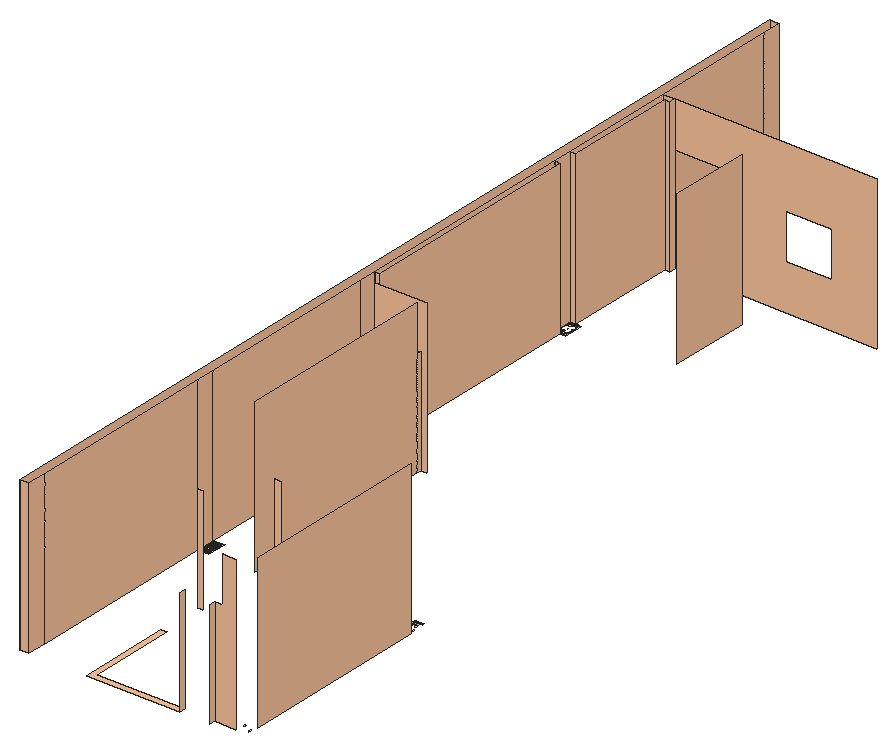
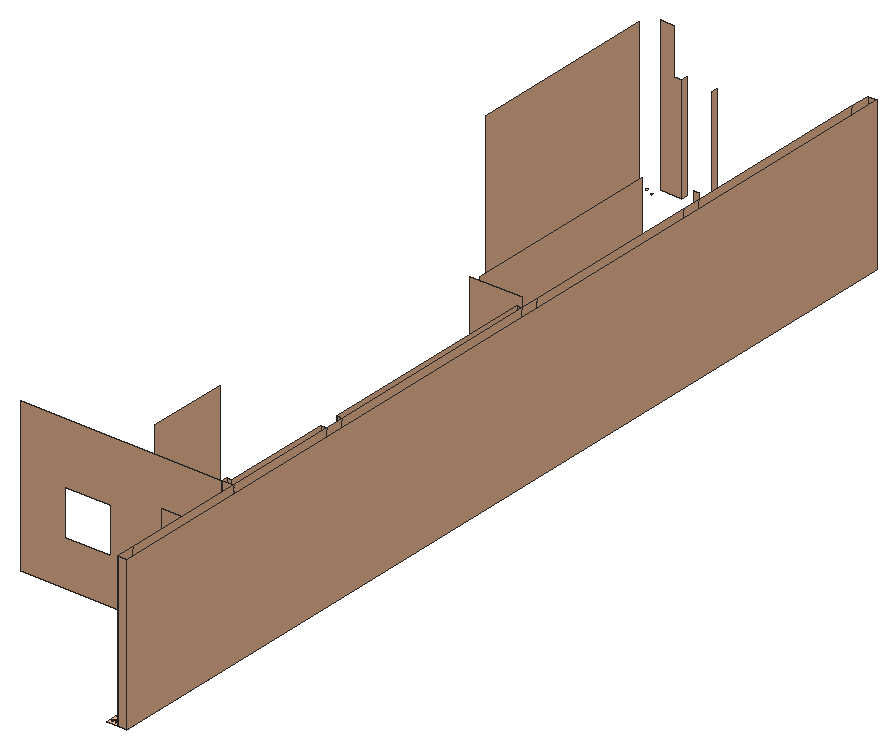
# SketchUp Ruby script. Lengths in inches.
U = 1.inch
M = Sketchup.active_model
def pt(a) = Geom::Point3d.new(a.map { |v| v * U })
def face(e, loops, mat)
  f = e.add_face(loops[0].map { |a| pt(a) })
  loops[1..].each { |l| e.add_face(l.map { |a| pt(a) }).erase! }
  f.material = f.back_material = mat if mat
  f
end
# faces: each face lists its corners as indices into pts; further lists are holes
def faces(e, pts, list, mat = nil) = list.each { |f| face(e, (f[0].is_a?(Array) ? f : [f]).map { |l| l.map { |i| pts[i] } }, mat) }
# xy, xz, yz: faces in a plane at the given z, y or x. An outline is a flat list of corners, or four numbers for a rectangle; further outlines are holes
def ring(l) = l.size == 4 ? [[l[0], l[1]], [l[2], l[1]], [l[2], l[3]], [l[0], l[3]]] : l.each_slice(2).to_a
def flat(e, list, mat, &to3) = list.each { |f| face(e, (f[0].is_a?(Array) ? f : [f]).map { |l| ring(l).map { |u, v| to3.(u, v) } }, mat) }
def xy(e, z, list, mat = nil) = flat(e, list, mat) { |x, y| [x, y, z] }
def xz(e, y, list, mat = nil) = flat(e, list, mat) { |x, z| [x, y, z] }
def yz(e, x, list, mat = nil) = flat(e, list, mat) { |y, z| [x, y, z] }
def lines(e, pts, list) = list.each { |a, b| e.add_line(pt(pts[a]), pt(pts[b])) }
# prism: a flat outline (further loops are holes) pulled along v
def prism(e, loops, v, mat = nil)
  f = face(e, loops, mat); d = Geom::Vector3d.new(v.map { |x| x * U })
  f.pushpull(f.normal.samedirection?(d) ? d.length : -d.length)
end
def box(e, o, s, mat = nil) = prism(e, [[o, [o[0] + s[0], o[1], o[2]], [o[0] + s[0], o[1] + s[1], o[2]], [o[0], o[1] + s[1], o[2]]]], [0, 0, s[2]], mat)
def at(x, y, z, deg = 0) = Geom::Transformation.translation(pt([x, y, z])) * Geom::Transformation.rotation(ORIGIN, Z_AXIS, deg.degrees)
def axes(o, x, y, z) = Geom::Transformation.new([*x, 0, *y, 0, *z, 0, *pt(o).to_a, 1])
def part(name) = M.definitions.add(name)
# library, detail: a bought-in or finely detailed component or shape, given as its bounding box
def library(name, o, s) = part(name).tap { |d| box(d.entities, o, s) }
def detail(e, o, s) = box(e.add_group.entities, o, s)
def put(e, d, t, mat = nil) = e.add_instance(d, t).tap { |i| i.material = mat if mat }
def group(e, t, mat = nil) = e.add_group.tap { |g| g.transformation = t; g.material = mat if mat }.entities
root = M.entities
M.materials.add("[Color A02]1").color = [252, 197, 157]
xy(root,131.89,[[0.9,46.0625,7.87,784.43],[52.9375,46.0625,52.9375,119.63,57.37,119.63,57.37,50.62,126.53,50.62,126.53,46.0625],[174.69,53.72,174.88,53.91,174.88,55.31,174.69,55.49,173.8125,54.6],[174.88,55.31,174.88,55.6875,174.69,55.49],[167.91,57.46,168.55,58.09,167.91,58.73],
  [[7.87,212.2,16.86,227.14],[8.88,213.21,15.84,226.13]],[8.88,213.21,9.13,213.21,9.51,213.59,8.88,214.22],[9.13,213.21,9.89,213.21,9.51,213.59],[9.89,213.21,10.9,213.21,11.28,213.59,10.4,214.48,9.51,213.59],[10.9,213.21,11.66,213.21,11.28,213.59],
  [11.66,213.21,12.68,213.21,13.06,213.59,12.17,214.48,11.28,213.59],[12.68,213.21,13.4375,213.21,13.06,213.59],[13.4375,213.21,14.45,213.21,14.83,213.59,13.94,214.48,13.06,213.59],[14.45,213.21,15.21,213.21,14.83,213.59],[15.21,213.21,15.84,213.21,15.84,214.22,15.65,214.42,14.83,213.59],
  [168.17,213.21,168.93,213.21,168.55,213.59],[9.51,213.59,10.4,214.48,9.51,215.36,8.88,214.73,8.88,214.22],[11.28,213.59,12.17,214.48,11.28,215.36,10.4,214.48],[13.06,213.59,13.94,214.48,13.06,215.36,12.17,214.48],[14.83,213.59,15.65,214.42,14.78,215.3125,13.94,214.48],
  [15.84,214.22,15.84,214.6,15.65,214.42],[174.88,214.22,174.88,214.6,174.69,214.42],[15.65,214.42,15.84,214.6,15.84,216,15.65,216.1875,14.78,215.3125],[174.69,214.42,174.88,214.6,174.88,216,174.69,216.1875,173.8125,215.3125],[10.4,214.48,11.28,215.36,10.4,216.25,9.51,215.36],
  [12.17,214.48,13.06,215.36,12.17,216.25,11.28,215.36],[13.94,214.48,14.78,215.3125,13.9,216.21,13.06,215.36],[8.88,214.73,9.51,215.36,8.88,216],[14.78,215.3125,15.65,216.1875,14.78,217.08,13.9,216.21],[9.51,215.36,10.4,216.25,9.51,217.14,8.88,216.5,8.88,216],
  [11.28,215.36,12.17,216.25,11.28,217.14,10.4,216.25],[13.06,215.36,13.9,216.21,13.02,217.1,12.17,216.25],[15.84,216,15.84,216.38,15.65,216.1875],[15.65,216.1875,15.84,216.38,15.84,217.77,15.65,217.96,14.78,217.08],[13.9,216.21,14.78,217.08,13.9,217.98,13.02,217.1],
  [10.4,216.25,11.28,217.14,10.4,218.02,9.51,217.14],[12.17,216.25,13.02,217.1,12.14,217.99,11.28,217.14],[8.88,216.5,9.51,217.14,8.88,217.77],[168.04,216.63,169.05,216.63,168.55,217.14],[14.78,217.08,15.65,217.96,14.77,218.85,13.9,217.98],
  [13.02,217.1,13.9,217.98,13.02,218.87,12.14,217.99],[9.51,217.14,10.4,218.02,9.51,218.91,8.88,218.28,8.88,217.77],[11.28,217.14,12.14,217.99,11.26,218.89,10.4,218.02],[15.84,217.77,15.84,218.15,15.65,217.96],[15.65,217.96,15.84,218.15,15.84,219.54,15.65,219.73,14.77,218.85],
  [13.9,217.98,14.77,218.85,13.88,219.73,13.02,218.87],[12.14,217.99,13.02,218.87,12.14,219.77,11.26,218.89],[10.4,218.02,11.26,218.89,10.38,219.78,9.51,218.91],[169.43,218.02,170.3,218.89,169.42,219.78,168.55,218.91],[8.88,218.28,9.51,218.91,8.88,219.54],
  [14.77,218.85,15.65,219.73,14.77,220.62,13.88,219.73],[13.02,218.87,13.88,219.73,12.99,220.62,12.14,219.77],[11.26,218.89,12.14,219.77,11.26,220.66,10.38,219.78],[9.51,218.91,10.38,219.78,9.51,220.67,8.88,220.05,8.88,219.54],[168.55,218.91,169.42,219.78,168.55,220.67,167.91,220.05,167.91,219.54],
  [15.84,219.54,15.84,219.92,15.65,219.73],[13.88,219.73,14.77,220.62,13.88,221.51,12.99,220.62],[15.65,219.73,15.84,219.92,15.84,221.32,15.65,221.51,14.77,220.62],[172.92,219.73,173.8,220.62,172.92,221.51,172.03,220.62],[12.14,219.77,12.99,220.62,12.11,221.51,11.26,220.66],
  [10.38,219.78,11.26,220.66,10.4,221.54,9.51,220.67],[169.42,219.78,170.3,220.66,169.44,221.54,168.55,220.67],[8.88,220.05,9.51,220.67,8.88,221.32],[167.91,220.05,168.55,220.67,167.91,221.32],[12.99,220.62,13.88,221.51,12.99,222.39,12.11,221.51],
  [14.77,220.62,15.65,221.51,14.77,222.39,13.88,221.51],[11.26,220.66,12.11,221.51,11.25,222.37,10.4,221.54],[9.51,220.67,10.4,221.54,9.51,222.44,8.88,221.82,8.88,221.32],[168.55,220.67,169.44,221.54,168.55,222.44,167.91,221.82,167.91,221.32],[15.84,221.32,15.84,221.7,15.65,221.51],
  [12.11,221.51,12.99,222.39,12.14,223.25,11.25,222.37],[13.88,221.51,14.77,222.39,13.88,223.28,12.99,222.39],[15.65,221.51,15.84,221.7,15.84,223.09,15.65,223.28,14.77,222.39],[10.4,221.54,11.25,222.37,10.36,223.26,9.51,222.44],[8.88,221.82,9.51,222.44,8.88,223.09],
  [170.28,222.37,171.18,223.25,170.29,224.13,169.39,223.26],[12.99,222.39,13.88,223.28,13.04,224.12,12.14,223.25],[14.77,222.39,15.65,223.28,14.77,224.16,13.88,223.28],[172.03,222.39,172.92,223.28,172.07,224.12,171.33,223.4,171.33,223.09],[9.51,222.44,10.36,223.26,9.46,224.15,8.88,223.6,8.88,223.09],
  [168.55,222.44,169.39,223.26,168.5,224.15,167.91,223.6,167.91,223.09],[15.84,223.09,15.84,223.47,15.65,223.28],[12.14,223.25,13.04,224.12,12.15,225,11.26,224.13],[10.36,223.26,11.26,224.13,10.37,225.02,9.46,224.15],[13.88,223.28,14.77,224.16,13.93,225,13.04,224.12],
  [171.33,223.4,172.07,224.12,171.33,224.86],[8.88,223.6,9.46,224.15,8.88,224.73],[13.04,224.12,13.93,225,13.05,225.88,12.15,225],[11.26,224.13,12.15,225,11.28,225.88,10.37,225.02],[170.29,224.13,171.19,225,170.3125,225.88,169.41,225.02],
  [9.46,224.15,10.37,225.02,9.49,225.89,8.88,225.37,8.88,224.73],[14.77,224.16,15.65,225.05,14.83,225.875,13.93,225],[12.15,225,13.05,225.88,12.8,226.13,11.54,226.13,11.28,225.88],[13.93,225,14.83,225.875,14.58,226.13,13.31,226.13,13.05,225.88],[172.97,225,173.86,225.875,173.61,226.13,172.35,226.13,172.09,225.88],
  [10.37,225.02,11.28,225.88,11.03,226.13,9.76,226.13,9.49,225.89],[15.65,225.05,15.84,225.24,15.84,226.13,15.08,226.13,14.83,225.875],[174.6875,225.05,174.88,225.24,174.88,226.13,174.12,226.13,173.86,225.875],[171.33,225.14,172.09,225.88,171.84,226.13,171.33,226.13],[8.88,225.37,9.49,225.89,9.26,226.13,8.88,226.13],
  [167.91,225.37,168.53,225.89,168.29,226.13,167.91,226.13],[14.83,225.875,15.08,226.13,14.58,226.13],[11.28,225.88,11.54,226.13,11.03,226.13],[13.05,225.88,13.31,226.13,12.8,226.13],[9.49,225.89,9.76,226.13,9.26,226.13],
  [7.87,371.24,12.42,371.24,12.42,372.26,8.88,372.26,8.88,385.3,12.42,385.3,12.42,386.1875,7.87,386.1875],[12.42,371.24,16.86,371.24,16.86,386.1875,12.42,386.1875,12.42,385.3,15.84,385.3,15.84,372.26,12.42,372.26],[9.51,372.64,10.4,373.52,9.51,374.41,8.88,373.78,8.88,373.27],[13.02,376.14,13.9,377.02,13.02,377.92,12.42,377.32,12.42,376.75],[12.42,376.75,12.42,377.32,12.14,377.04],
  [15.84,376.82,15.84,377.19,15.65,377.01],[12.42,378.52,12.42,379.09,12.14,378.8125],[15.84,378.59,15.84,378.97,15.65,378.78],[13.02,379.69,13.9,380.57,13.02,381.46,12.42,380.87,12.42,380.3],[11.26,379.71,12.14,380.58,11.26,381.48,10.38,380.6],
  [12.42,380.3,12.42,380.87,12.14,380.58],[15.84,380.36,15.84,380.74,15.66,380.55],[15.66,380.55,15.84,380.74,15.84,382.13,15.66,382.33,14.78,381.45],[10.38,380.6,11.26,381.48,10.38,382.37,9.51,381.49],[8.88,380.87,9.51,381.49,8.88,382.13],
  [12.42,380.87,13.02,381.46,12.42,382.07],[11.26,381.48,12.14,382.36,11.27,383.25,10.38,382.37],[9.51,381.49,10.38,382.37,9.51,383.27,8.88,382.64,8.88,382.13],[15.84,382.13,15.84,382.51,15.66,382.33],[8.88,382.64,9.51,383.27,8.88,383.91],
  [15.84,383.91,15.84,384.29,15.66,384.11],[14.82,385.03,15.08,385.3,14.58,385.3],[9.51,385.04,9.76,385.3,9.26,385.3],[11.28,385.04,11.54,385.3,11.03,385.3],[13.05,385.04,13.31,385.3,12.8,385.3],
  [7.87,563.34,12.42,563.34,12.42,564.35,8.88,564.35,8.88,577.27,12.42,577.27,12.42,578.28,7.87,578.28],[12.42,563.34,16.86,563.34,16.86,578.28,12.42,578.28,12.42,577.27,15.84,577.27,15.84,564.35,12.42,564.35],[15.21,564.35,15.84,564.35,15.84,565.36,15.65,565.56,14.83,564.73],[14.83,564.73,15.65,565.56,14.78,566.45,13.94,565.62],[12.42,565.36,12.42,565.87,12.17,565.62],
  [15.84,565.36,15.84,565.74,15.65,565.56],[15.65,565.56,15.84,565.74,15.84,567.14,15.65,567.33,14.78,566.45],[10.4,565.62,11.28,566.5,10.4,567.39,9.51,566.5],[12.17,565.62,12.42,565.87,12.42,567.14,12.17,567.39,11.28,566.5],[11.28,566.5,12.17,567.39,11.28,568.28,10.4,567.39],
  [12.42,567.14,12.42,567.64,12.17,567.39],[15.84,567.14,15.84,567.52,15.65,567.33],[15.84,568.91,15.84,569.29,15.65,569.1],[12.42,570.56,12.42,571.1875,12.11,570.87],[15.84,570.68,15.84,571.0625,15.65,570.87],
  [15.65,570.87,15.84,571.0625,15.84,572.46,15.65,572.65,14.77,571.76],[15.84,572.46,15.84,572.84,15.65,572.65],[15.84,574.23,15.84,574.61,15.65,574.42],[10.36,574.4,11.26,575.27,10.37,576.16,9.46,575.29],[8.88,574.73,9.46,575.29,8.88,575.875],
  [11.26,575.27,12.15,576.14,11.28,577.02,10.37,576.16],[9.46,575.29,10.37,576.16,9.49,577.03,8.88,576.51,8.88,575.875],[12.42,575.875,12.42,576.41,12.15,576.14],[15.84,576,15.84,576.38,15.65,576.19],[12.15,576.14,12.42,576.41,12.42,577.27,11.54,577.27,11.28,577.02],
  [10.37,576.16,11.28,577.02,11.03,577.27,9.76,577.27,9.49,577.03],[15.65,576.19,15.84,576.38,15.84,577.27,15.08,577.27,14.83,577.02],[12.42,576.41,13.05,577.02,12.8,577.27,12.42,577.27],[8.88,576.51,9.49,577.03,9.26,577.27,8.88,577.27],[11.28,577.02,11.54,577.27,11.03,577.27],
  [13.05,577.02,13.31,577.27,12.8,577.27],[14.83,577.02,15.08,577.27,14.58,577.27],[9.49,577.03,9.76,577.27,9.26,577.27],[7.87,578.28,7.87,670.34,16.86,670.34,16.86,665.91,12.42,665.91,12.42,578.28],[[7.87,769.36,16.86,784.43],[11.28,781.39,10.4,782.28,9.51,783.16,9.26,783.42,13.31,783.42,13.05,783.16,12.8,783.42,11.54,783.42,11.28,783.16,11.03,783.42,9.76,783.42,9.51,783.16,10.4,782.28,11.28,783.16,12.17,782.28],[10.4,773.41,9.51,774.3,10.4,775.1875,11.28,774.3],[12.17,776.96,11.28,777.85,12.17,778.73,13.06,777.85],[10.4,775.1875,9.51,776.07,10.4,776.96,11.28,776.07],[13.94,778.73,13.06,779.62,13.94,780.51,14.83,779.62],[10.4,776.96,9.51,777.85,10.4,778.73,11.28,777.85],[12.17,775.1875,11.28,776.07,12.17,776.96,13.06,776.07],[13.92,771.67,13.03,772.56,13.91,773.45,14.79,772.57],[13.94,780.51,13.06,781.39,13.92,782.25,14.79,781.35],[14.78,774.35,13.94,775.1875,14.83,776.07,15.66,775.25],[15.66,782.22,14.82,783.15,15.08,783.42,15.84,783.42,15.84,782.4],[8.88,780.76,8.88,782.02,9.51,781.39]],
  [8.88,770.375,9.13,770.375,9.51,770.75,8.88,771.39],[9.89,770.375,10.9,770.375,11.28,770.76,10.4,771.64,9.51,770.75],[11.66,770.375,12.68,770.375,13.05,770.76,12.15,771.66,11.28,770.76],[12.68,770.375,13.4375,770.375,13.05,770.76,13.92,771.67,14.8125,770.77,15.66,771.7,14.79,772.57,13.92,771.67,13.03,772.56,12.15,771.66,13.05,770.76],[13.4375,770.375,14.45,770.375,14.8125,770.77,13.92,771.67,13.05,770.76],
  [10.4,771.64,11.28,772.53,12.17,773.41,13.06,774.3,13.91,773.45,13.03,772.56,12.17,773.41,11.28,772.53,10.4,773.41,9.51,772.53],[13.92,771.67,14.79,772.57,13.91,773.45,13.03,772.56],[8.88,771.89,9.51,772.53,8.88,773.16],[13.03,772.56,13.91,773.45,13.06,774.3,12.17,773.41],[14.79,772.57,15.66,773.47,14.78,774.35,13.91,773.45],
  [10.4,773.41,11.28,774.3,10.4,775.1875,9.51,774.3],[12.17,773.41,13.06,774.3,12.17,775.1875,11.28,774.3],[8.88,773.67,9.51,774.3,8.88,774.93],[14.78,774.35,15.66,775.25,14.83,776.07,13.94,775.1875],[10.4,775.1875,11.28,776.07,10.4,776.96,9.51,777.85,10.4,778.73,11.28,777.85,12.17,778.73,11.28,779.62,10.4,778.73,11.28,777.85,10.4,776.96,9.51,776.07],
  [12.17,775.1875,13.06,776.07,12.17,776.96,11.28,776.07],[8.88,775.44,9.51,776.07,8.88,776.71],[10.4,776.96,11.28,777.85,10.4,778.73,9.51,777.85],[8.88,777.21,9.51,777.85,8.88,778.48],[12.17,778.73,13.06,779.62,12.17,780.51,11.28,779.62],
  [13.94,778.73,14.83,779.62,13.94,780.51,13.06,779.62],[11.28,779.62,12.17,780.51,11.28,781.39,10.4,780.51],[14.83,779.62,15.66,780.45,14.79,781.35,13.94,780.51],[13.94,780.51,14.79,781.35,13.92,782.25,13.06,781.39],[11.28,781.39,12.17,782.28,11.28,783.16,10.4,782.28]],"[Color A02]1")
xz(root,46.0625,[[0.9,131.89,7.87,251.89]],"[Color A02]1")
xz(root,50.62,[[150.53,131.89,150.53,215.89,156.53,215.89,156.53,251.89,166.9,251.89,166.9,131.89]],"[Color A02]1")
xz(root,155.6,[[52.9375,131.89,57.37,215.89]],"[Color A02]1")
xz(root,194.22,[[82.95,131.89,87.38,215.89]],"[Color A02]1")
xz(root,375.68,[[52.9375,131.89,52.9375,215.89,16.86,215.89,16.86,251.89,57.37,251.89,57.37,131.89]],"[Color A02]1")
xz(root,386.1875,[[7.87,131.89,12.42,251.89]],"[Color A02]1")
xz(root,563.34,[[7.87,131.89,12.42,251.89]],"[Color A02]1")
xz(root,578.28,[[7.87,131.89,12.42,251.89]],"[Color A02]1")
xz(root,665.91,[[12.42,131.89,16.86,251.89]],"[Color A02]1")
xz(root,670.34,[[7.87,131.89,16.86,251.89],[[64.84,131.89,64.84,215.89,16.86,215.89,16.86,251.89,175.89,251.89,175.89,131.89],[104.48,167.89,140.48,203.89]]],"[Color A02]1")
xz(root,784.43,[[0.9,131.89,7.87,251.89]],"[Color A02]1")
yz(root,0.9,[[46.0625,131.89,784.43,251.89]],"[Color A02]1")
yz(root,7.87,[[46.0625,131.89,61.13,251.89],[61.13,131.89,212.2,251.89],[212.2,131.89,227.14,251.89],[227.14,131.89,371.24,251.89],[371.24,131.89,386.1875,251.89],
  [386.1875,131.89,563.34,251.89],[563.34,131.89,578.28,251.89],[578.28,131.89,670.34,251.89],[670.34,131.89,769.36,251.89],[769.36,131.89,784.43,251.89]],"[Color A02]1")
yz(root,12.42,[[386.1875,131.89,563.34,251.89],[578.28,131.89,665.91,251.89]],"[Color A02]1")
yz(root,16.86,[[665.91,131.89,670.34,251.89]],"[Color A02]1")
yz(root,52.9375,[[212.2,131.89,371.24,251.89],[371.24,131.89,375.68,215.89]],"[Color A02]1")
yz(root,92.44,[[578.28,131.89,641.85,251.89]],"[Color A02]1")
yz(root,126.53,[[46.0625,131.89,50.62,215.89]],"[Color A02]1")
yz(root,150.53,[[46.0625,131.89,50.62,215.89]],"[Color A02]1")
yz(root,175.89,[[61,131.89,212.21,251.89]],"[Color A02]1")
